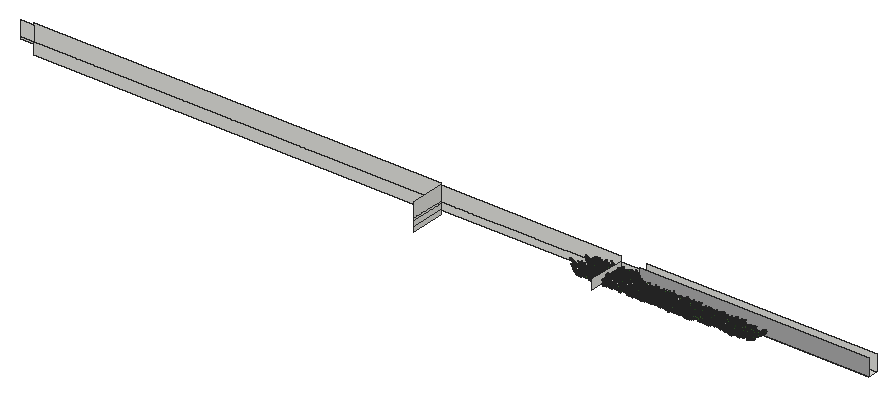
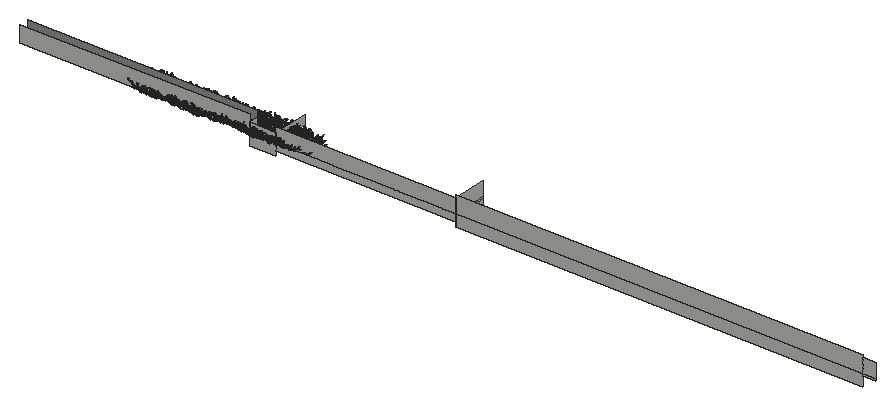
# SketchUp Ruby script. Lengths in inches.
U = 1.inch
M = Sketchup.active_model
def pt(a) = Geom::Point3d.new(a.map { |v| v * U })
def face(e, loops, mat)
  f = e.add_face(loops[0].map { |a| pt(a) })
  loops[1..].each { |l| e.add_face(l.map { |a| pt(a) }).erase! }
  f.material = f.back_material = mat if mat
  f
end
# faces: each face lists its corners as indices into pts; further lists are holes
def faces(e, pts, list, mat = nil) = list.each { |f| face(e, (f[0].is_a?(Array) ? f : [f]).map { |l| l.map { |i| pts[i] } }, mat) }
# xy, xz, yz: faces in a plane at the given z, y or x. An outline is a flat list of corners, or four numbers for a rectangle; further outlines are holes
def ring(l) = l.size == 4 ? [[l[0], l[1]], [l[2], l[1]], [l[2], l[3]], [l[0], l[3]]] : l.each_slice(2).to_a
def flat(e, list, mat, &to3) = list.each { |f| face(e, (f[0].is_a?(Array) ? f : [f]).map { |l| ring(l).map { |u, v| to3.(u, v) } }, mat) }
def xy(e, z, list, mat = nil) = flat(e, list, mat) { |x, y| [x, y, z] }
def xz(e, y, list, mat = nil) = flat(e, list, mat) { |x, z| [x, y, z] }
def yz(e, x, list, mat = nil) = flat(e, list, mat) { |y, z| [x, y, z] }
def lines(e, pts, list) = list.each { |a, b| e.add_line(pt(pts[a]), pt(pts[b])) }
# prism: a flat outline (further loops are holes) pulled along v
def prism(e, loops, v, mat = nil)
  f = face(e, loops, mat); d = Geom::Vector3d.new(v.map { |x| x * U })
  f.pushpull(f.normal.samedirection?(d) ? d.length : -d.length)
end
def box(e, o, s, mat = nil) = prism(e, [[o, [o[0] + s[0], o[1], o[2]], [o[0] + s[0], o[1] + s[1], o[2]], [o[0], o[1] + s[1], o[2]]]], [0, 0, s[2]], mat)
def at(x, y, z, deg = 0) = Geom::Transformation.translation(pt([x, y, z])) * Geom::Transformation.rotation(ORIGIN, Z_AXIS, deg.degrees)
def axes(o, x, y, z) = Geom::Transformation.new([*x, 0, *y, 0, *z, 0, *pt(o).to_a, 1])
def part(name) = M.definitions.add(name)
# library, detail: a bought-in or finely detailed component or shape, given as its bounding box
def library(name, o, s) = part(name).tap { |d| box(d.entities, o, s) }
def detail(e, o, s) = box(e.add_group.entities, o, s)
def put(e, d, t, mat = nil) = e.add_instance(d, t).tap { |i| i.material = mat if mat }
def group(e, t, mat = nil) = e.add_group.tap { |g| g.transformation = t; g.material = mat if mat }.entities
root = M.entities
M.materials.add("Material82").color = [68, 110, 58]
M.materials.add("Material83").color = [48, 90, 38]
M.materials.add("Material84").color = [68, 110, 48]
M.materials.add("Material85").color = [48, 90, 48]
M.materials.add("Material86").color = [58, 110, 58]
M.materials.add("Material87").color = [58, 90, 38]
M.materials.add("Material88").color = [68, 100, 58]
M.materials.add("Material89").color = [48, 100, 38]
M.materials.add("[Color M03]1").color = [170, 170, 170]
c1 = part("grass00")
p = [[-0.6875,0.15,0],[-0.56,0.08,5.52],[-0.04,0.03,2.76],[0.48,-0.02,0],[0.35,-0.02,5.52],[-0.1,-0.14,5.52],
  [-0.12,0.65,8.37],[-0.42,0.65,8.37]]
faces(c1.entities,p,[[0,1,2,3],[3,2,4],[1,5,2],[5,4,2],[1,6,5],[4,5,6],[7,6,1]])
c2 = part("Group16\#1")
put(c2.entities,c1,axes([1.44,-0.61,-0.01],[0.05352,0.12609,0],[-0.10704,0.04543,0.07239],[0.06664,-0.02828,0.11628]),"Material85")
put(c2.entities,c1,axes([0.76,-0.15,-0.01],[0.04676,0.24062,0],[-0.23162,0.04501,0.06642],[0.0652,-0.01267,0.23595]),"Material82")
put(c2.entities,c1,axes([0.79,0.01,-0.01],[-0.00606,0.34651,0],[-0.34381,-0.00602,0.0432],[0.04319,0.00076,0.34386]))
put(c2.entities,c1,axes([1,0.23,-0.01],[-0.07192,0.31144,0],[-0.28722,-0.06632,0.1236],[0.12043,0.02781,0.29478]),"Material84")
put(c2.entities,c1,axes([1.66,0.77,-0.01],[-0.13828,0.29651,0],[-0.21551,-0.1005,0.22471],[0.20365,0.09498,0.23779]),"Material89")
put(c2.entities,c1,axes([0.6875,0.52,-0.01],[-0.18126,0.24051,0],[-0.22746,-0.17142,0.09788],[0.07817,0.05891,0.28481]),"Material84")
put(c2.entities,c1,axes([0.68,0.78,-0.01],[-0.215,0.18688,0],[-0.12385,-0.14248,0.21334],[0.13995,0.16101,0.18878]),"Material82")
put(c2.entities,c1,axes([0.56,1,-0.01],[-0.13756,0.07624,0],[-0.06159,-0.11112,0.0927],[0.04494,0.08108,0.12705]),"Material84")
put(c2.entities,c1,axes([0.2,0.64,-0.01],[-0.23729,0.07254,0],[-0.05711,-0.18681,0.153],[0.04473,0.14632,0.19535]),"Material89")
put(c2.entities,c1,axes([0.0625,0.72,-0.01],[-0.28874,0.02525,0],[-0.02179,-0.24916,0.14647],[0.01276,0.14591,0.25012]),"Material82")
put(c2.entities,c1,axes([-0.08,0.62,-0.01],[-0.34089,-0.04187,0],[0.03255,-0.26504,0.216],[-0.02633,0.21439,0.26703]),"Material89")
put(c2.entities,c1,axes([-0.34,0.98,-0.01],[-0.14314,-0.0493,0],[0.04397,-0.12769,0.06843],[-0.02228,0.0647,0.13505]),"Material89")
put(c2.entities,c1,axes([-0.87,1.45,-0.01],[-0.23488,-0.14114,0],[0.13761,-0.22901,0.06087],[-0.03135,0.05217,0.26717]))
put(c2.entities,c1,axes([-0.72,0.77,-0.01],[-0.14208,-0.13251,0],[0.07209,-0.0773,0.16301],[-0.11118,0.11922,0.1057]),"Material89")
put(c2.entities,c1,axes([-0.62,0.43,-0.01],[-0.14845,-0.21203,0],[0.18654,-0.13061,0.12304],[-0.10079,0.07057,0.22772]),"Material82")
put(c2.entities,c1,axes([-0.68,0.29,-0.01],[-0.13639,-0.32136,0],[0.31723,-0.13464,0.05579],[-0.05136,0.0218,0.34462]),"Material83")
put(c2.entities,c1,axes([-0.64,0.125,-0.01],[-0.0458,-0.23569,0],[0.22124,-0.043,0.08276],[-0.08124,0.01579,0.22538]),"Material86")
put(c2.entities,c1,axes([-1.6,-0.03,-0.01],[0.00576,-0.32897,0],[0.27526,0.00482,0.18018],[-0.18015,-0.00315,0.2753]),"Material84")
put(c2.entities,c1,axes([-1.36,-0.31,-0.01],[0.05718,-0.24765,0],[0.18172,0.04196,0.17267],[-0.16825,-0.03885,0.1865]),"Material89")
put(c2.entities,c1,axes([-1.54,-0.72,-0.01],[0.06537,-0.14017,0],[0.13555,0.06321,0.03939],[-0.0357,-0.01665,0.14956]))
put(c2.entities,c1,axes([-1.19,-0.9,-0.01],[0.09597,-0.12735,0],[0.11214,0.08451,0.07557],[-0.06035,-0.04548,0.14042]),"Material88")
put(c2.entities,c1,axes([-0.47,-0.54,-0.01],[0.11588,-0.10072,0],[0.0618,0.0711,0.12124],[-0.07953,-0.0915,0.0942]))
put(c2.entities,c1,axes([-0.47,-0.84,-0.01],[0.11927,-0.0661,0],[0.06603,0.11913,0.00646],[-0.00313,-0.00565,0.13621]),"Material84")
put(c2.entities,c1,axes([-0.38,-1.24,-0.01],[0.28037,-0.08571,0],[0.0618,0.20215,0.20315],[-0.05939,-0.19428,0.21139]),"Material88")
put(c2.entities,c1,axes([-0.06,-0.66,-0.01],[0.22719,-0.01987,0],[0.01247,0.14255,0.17758],[-0.01547,-0.17691,0.1431]),"Material87")
put(c2.entities,c1,axes([0.11,-0.89,-0.01],[0.14882,0.01828,0],[-0.01058,0.08611,0.12229],[0.01491,-0.12138,0.08676]),"Material85")
put(c2.entities,c1,axes([0.25,-0.72,-0.01],[0.20481,0.07053,0],[-0.06206,0.18022,0.10291],[0.03351,-0.0973,0.1906]),"Material85")
put(c2.entities,c1,axes([0.85,-1.42,-0.01],[0.16481,0.09904,0],[-0.09472,0.15762,0.05616],[0.02893,-0.04814,0.18389]),"Material84")
put(c2.entities,c1,axes([1.01,-1.09,-0.01],[0.21858,0.20385,0],[-0.17495,0.1876,0.15339],[0.10462,-0.11218,0.25652]),"Material89")
put(c2.entities,c1,axes([1.01,-0.71,-0.01],[0.08733,0.12473,0],[-0.06445,0.04512,0.13037],[0.1068,-0.07477,0.07867]),"Material85")
c3 = part("Group15\#1")
put(c3.entities,c2,at(0,0,0))
c4 = part("3darcstudiotree_grass00\#1")
put(c4.entities,c3,at(0,0,0))
xy(root,-34.17,[[1674.99,381.72,1831.09,387.84]])
xz(root,381.72,[[1674.99,-34.17,1831.09,-22.8]],"[Color M03]1")
xz(root,387.84,[[1257.22,-42.1875,1534.73,-34.17],[1657.41,-42.1875,1674.99,-34.17],[1534.73,-39.125,1657.41,-34.17],[1248.34,-35.625,1257.22,-34.17],[1248.34,-34.17,1257.22,-24.25],
  [1257.22,-34.17,1534.73,-22.8],[1534.73,-34.17,1657.41,-24.25],[1657.41,-34.17,1674.99,-27.66],[1674.99,-34.17,1831.09,-22.8]])
yz(root,1534.73,[[364.46,-42.1875,387.84,-39.125],[364.46,-39.125,387.84,-35.625],[364.46,-35.625,387.84,-34.17],[364.46,-34.17,387.84,-24.25]])
yz(root,1657.41,[[362.97,-34.17,387.84,-27.66]])
yz(root,1674.99,[[381.72,-34.17,387.84,-27.66]])
put(root,c4,axes([1646.16,372.86,-34.17],[0.43217,-1.5656,0],[4.20709,0.18062,-0.01362],[0.0661,0.00284,1.54899]))
put(root,c4,axes([1667,373.03,-34.17],[0.37423,-1.77165,0],[3.6892,0.1212,-0.04948],[0.31334,0.01029,1.76318]))
put(root,c4,axes([1660.48,373.13,-34.17],[2.99211,-0.88341,0],[2.54027,1.33816,-0.01707],[0.06311,0.03325,1.96039]))
put(root,c4,axes([1700.4,372.41,-34.17],[-4.26886,-0.01451,0],[0.03771,-1.72573,-0.00939],[0.00047,-0.02147,1.9024]))
put(root,c4,axes([1689.54,372.79,-34.17],[3.91894,1.05311,0],[-2.36552,1.3691,-0.06012],[-0.14517,0.08402,1.3502]))
put(root,c4,axes([1681.87,373.13,-34.17],[3.33812,-0.00931,0],[0.03014,1.68097,-0.0442],[0.00131,0.07293,1.33678]))
put(root,c4,axes([1655.42,373.02,-34.17],[2.55431,1.01117,0],[-3.10398,1.2195,-0.03194],[-0.09397,0.03692,1.36388]))
put(root,c4,axes([1712.625,372.65,-34.17],[-3.78642,0.03695,0],[-0.11198,-1.78455,-0.01248],[-0.00125,-0.01991,1.37214]))
put(root,c4,axes([1744.15,372.82,-34.17],[-3.59063,0.36551,0],[-0.927,-1.41632,-0.03018],[-0.05381,-0.08221,1.98332]))
put(root,c4,axes([1716.72,372.76,-34.17],[-3.89357,0.61481,0],[-1.50479,-1.48217,-0.00598],[-0.01246,-0.01228,1.70205]))
put(root,c4,axes([1679.82,373.3125,-34.17],[-2.43659,-1.39628,0],[3.54139,-0.96116,-0.05298],[0.19991,-0.05426,1.4759]))
put(root,c4,axes([1670.83,373.45,-34.17],[2.25035,1.16277,0],[-2.68664,0.80868,-0.04536],[-0.27393,0.08245,1.92466]))
put(root,c4,axes([1720.54,374.24,-34.17],[0.94723,-1.59052,0],[4.2139,0.39031,-0.04288],[0.2193,0.02031,1.70449]))
put(root,c4,axes([1750.67,374.25,-34.17],[4.40385,0.48107,0],[-1.25638,1.78876,-0.02222],[-0.03253,0.04631,1.93436]))
put(root,c4,axes([1712.65,374.63,-34.17],[0.52677,-1.54843,0],[3.37532,0.17859,-0.00096],[0.0064,0.00034,1.71349]))
put(root,c4,axes([1655.41,374.65,-34.17],[1.00905,-1.48256,0],[4.12419,0.43657,-0.05256],[0.2523,0.02671,1.59089]))
put(root,c4,axes([1717.8125,374.45,-34.17],[-2.54975,-1.13663,0],[2.74994,-0.95943,-0.02762],[0.1264,-0.0441,1.68176]))
put(root,c4,axes([1703.84,374.86,-34.17],[4.10302,-0.30694,0],[0.8385,1.74326,-0.00778],[0.00611,0.0127,1.42033]))
put(root,c4,axes([1677.05,374.0625,-34.17],[-3.06856,1.30795,0],[-2.89535,-1.05647,-0.0352],[-0.142,-0.05181,1.62511]))
put(root,c4,axes([1689.47,374.78,-34.17],[0.60137,-1.69863,0],[3.35822,0.18491,-0.0384],[0.22932,0.01263,1.53253]))
put(root,c4,axes([1732.47,375.0625,-34.17],[3.06207,-0.55792,0],[1.42852,1.21938,-0.0238],[0.07482,0.06387,1.9133]))
put(root,c4,axes([1727.61,374.52,-34.17],[0.41076,1.77313,0],[-3.60416,0.12986,-0.02215],[-0.11578,0.00417,1.42375]))
put(root,c4,axes([1672.28,375.43,-34.17],[-0.12471,-1.80139,0],[4.72201,-0.05084,-0.06757],[0.3331,-0.00359,1.74608]))
put(root,c4,axes([1682.07,374.875,-34.17],[-0.2328,1.40639,0],[-3.78045,-0.09733,-0.01044],[-0.05523,-0.00142,1.50484]))
put(root,c4,axes([1744.24,374.77,-34.17],[-1.9685,1.46825,0],[-4.07305,-0.84931,-0.01892],[-0.07094,-0.01479,1.46501]))
put(root,c4,axes([1661.98,375.07,-34.17],[1.86247,1.54763,0],[-3.42195,0.64048,-0.01135],[-0.06523,0.01221,1.80626]))
put(root,c4,axes([1650.84,375.22,-34.17],[-0.22309,1.29668,0],[-4.38525,-0.11734,-0.00038],[-0.00168,-0.00004,1.44006]))
put(root,c4,axes([1737.04,375.41,-34.17],[1.22817,1.22832,0],[-3.29828,0.51292,-0.04901],[-0.28268,0.04396,1.64754]))
put(root,c4,axes([1697.9375,375.32,-34.17],[-0.96459,1.39728,0],[-4.50708,-0.48391,-0.06593],[-0.29103,-0.03125,1.60187]))
put(root,c4,axes([1696.28,375.42,-34.17],[0.06651,1.49398,0],[-4.62108,0.032,-0.00579],[-0.03066,0.00021,1.83497]))
put(root,c4,axes([1665.18,375.59,-34.17],[-3.98386,-0.59662,0],[1.47731,-1.53422,-0.04397],[0.0965,-0.10022,1.92843]))
put(root,c4,axes([1693.27,376.5,-34.17],[3.81628,-0.13918,0],[0.37321,1.59155,-0.00914],[0.00528,0.02252,1.90465]))
put(root,c4,axes([1664.96,376.41,-34.17],[3.87274,-0.73751,0],[1.55178,1.26734,-0.04306],[0.13654,0.11151,1.95064]))
put(root,c4,axes([1743.24,376.96,-34.17],[4.03419,0.29669,0],[-0.75311,1.59264,-0.00417],[-0.00465,0.00984,1.87295]))
put(root,c4,axes([1705.6,376.69,-34.17],[1.8424,1.14237,0],[-3.65624,0.91712,-0.00074],[-0.00371,0.00093,1.93092]))
put(root,c4,axes([1649.58,376.95,-34.17],[-2.10821,-1.47996,0],[3.50963,-0.77757,-0.0488],[0.18715,-0.04146,1.32723]))
put(root,c4,axes([1738.35,376.96,-34.17],[4.26727,0.66803,0],[-1.41698,1.40776,-0.04113],[-0.07249,0.07202,1.37498]))
put(root,c4,axes([1720.71,377.2,-34.17],[4.15464,-0.59094,0],[1.53872,1.68251,-0.06016],[0.09162,0.10018,1.52593]))
put(root,c4,axes([1716.68,376.61,-34.17],[0.64746,1.71828,0],[-3.59,0.21039,-0.03328],[-0.18561,0.01088,1.53387]))
put(root,c4,axes([1654.41,377.25,-34.17],[2.13524,-1.29449,0],[3.0122,0.77275,-0.01966],[0.10051,0.02579,1.64285]))
put(root,c4,axes([1689.64,376.78,-34.17],[-1.5249,1.25696,0],[-3.62628,-0.68422,-0.02774],[-0.1175,-0.02217,1.41462]))
put(root,c4,axes([1672.08,377.47,-34.17],[3.32502,-0.81851,0],[2.11953,1.33913,-0.03499],[0.11667,0.07371,1.88939]))
put(root,c4,axes([1645.69,376.76,-34.17],[-3.35215,0.96429,0],[-2.54913,-1.37823,-0.03459],[-0.11585,-0.06264,1.84283]))
put(root,c4,axes([1709.41,377.42,-34.17],[-1.38876,-1.54798,0],[3.56891,-0.49797,-0.03351],[0.18812,-0.02625,1.68972]))
put(root,c4,axes([1682.63,376.83,-34.17],[-1.7842,1.38137,0],[-4.14651,-0.83297,-0.01882],[-0.07173,-0.01441,1.49212]))
put(root,c4,axes([1728.79,377.7,-34.17],[0.96466,-1.81909,0],[3.32191,0.27398,-0.01603],[0.09156,0.00755,1.48463]))
put(root,c4,axes([1662.8125,377.27,-34.17],[-2.42169,0.94143,0],[-3.12641,-1.2508,-0.05994],[-0.19111,-0.07646,1.51606]))
put(root,c4,axes([1675.83,377.69,-34.17],[-1.63198,-1.29559,0],[3.66951,-0.7189,-0.01655],[0.08632,-0.01691,1.78815]))
put(root,c4,axes([1734.62,377.29,-34.17],[-1.97144,1.08801,0],[-3.33394,-0.93955,-0.01309],[-0.05439,-0.01533,1.56859]))
put(root,c4,axes([1750.06,377.8,-34.17],[-3.77025,-0.95024,0],[2.35793,-1.45505,-0.05584],[0.17762,-0.10961,1.93872]))
put(root,c4,axes([1700.46,377.51,-34.17],[-0.60649,1.78928,0],[-3.60415,-0.19,-0.04319],[-0.29403,-0.0155,1.87209]))
put(root,c4,axes([1717.27,378.77,-34.17],[2.12492,-1.52639,0],[3.32667,0.72027,-0.02765],[0.13101,0.02837,1.53783]))
put(root,c4,axes([1645.55,378.7,-34.17],[3.10066,0.47843,0],[-1.67535,1.68868,-0.03882],[-0.06401,0.06452,1.55956]))
put(root,c4,axes([1651.15,378.47,-34.17],[2.78968,1.01154,0],[-2.64,1.13236,-0.04265],[-0.18761,0.08047,1.90027]))
put(root,c4,axes([1660.72,378.8,-34.17],[4.11116,0.47333,0],[-1.05643,1.42708,-0.03197],[-0.04362,0.05892,1.37583]))
put(root,c4,axes([1688.89,378.72,-34.17],[3.33503,1.17525,0],[-2.6851,1.18507,-0.00121],[-0.00399,0.00176,1.48985]))
put(root,c4,axes([1722.43,379.08,-34.17],[2.11135,-1.17998,0],[3.12805,0.87051,-0.01427],[0.05324,0.01482,1.30992]))
put(root,c4,axes([1706.38,379,-34.17],[-2.24585,-1.17679,0],[2.75058,-0.81643,-0.02546],[0.1532,-0.04547,1.94365]))
put(root,c4,axes([1728.08,379.3,-34.17],[-1.90322,-1.23489,0],[2.93996,-0.70472,-0.04312],[0.27444,-0.06578,1.92045]))
put(root,c4,axes([1655.09,378.9,-34.17],[-2.52665,1.52426,0],[-3.1276,-0.80632,-0.05029],[-0.29899,-0.07708,1.98932]))
put(root,c4,axes([1699.92,378.94,-34.17],[-1.50368,1.17097,0],[-3.52829,-0.70467,-0.03106],[-0.12382,-0.02473,1.32443]))
put(root,c4,axes([1748.36,379.75,-34.17],[3.38929,-0.88137,0],[2.3631,1.41334,-0.02666],[0.06787,0.04059,1.48784]))
put(root,c4,axes([1711.625,379.73,-34.17],[2.20658,-1.37183,0],[2.86337,0.71632,-0.01781],[0.08885,0.02223,1.50117]))
put(root,c4,axes([1693.3125,379.64,-34.17],[0.14571,-1.35454,0],[4.55175,0.07615,-0.04061],[0.20314,0.0034,1.70991]))
put(root,c4,axes([1738.37,379.53,-34.17],[3.73542,0.56333,0],[-1.36375,1.40645,-0.02441],[-0.06005,0.06193,1.97124]))
put(root,c4,axes([1665.98,379.17,-34.17],[0.11998,1.39847,0],[-4.49149,0.05993,-0.06181],[-0.32467,0.00433,1.77032]))
put(root,c4,axes([1733.68,379.47,-34.17],[2.76774,0.7917,0],[-1.93345,1.05126,-0.02439],[-0.09329,0.05072,1.60766]))
put(root,c4,axes([1672.14,379.76,-34.17],[2.90846,1.13793,0],[-2.61613,1.03996,-0.02475],[-0.10205,0.04057,1.62992]))
put(root,c4,axes([1744.18,379.87,-34.17],[1.66114,1.62878,0],[-3.87747,0.61504,-0.0015],[-0.00686,0.00109,1.54039]))
put(root,c4,axes([1675.9375,379.91,-34.17],[0.65055,1.72425,0],[-3.43127,0.20135,-0.01524],[-0.11013,0.00646,1.90022]))
put(root,c4,axes([1684.6,379.91,-34.17],[-2.50108,0.95556,0],[-2.98511,-1.21518,-0.02879],[-0.10959,-0.04461,1.7592]))
put(root,c4,axes([1737.12,380.69,-34.17],[2.03121,-1.05332,0],[3.7313,1.11909,-0.04371],[0.13933,0.04179,1.40723]))
put(root,c4,axes([1672.25,380.76,-34.17],[4.3644,0.14123,0],[-0.27589,1.32601,-0.01884],[-0.00836,0.04017,1.37151]))
put(root,c4,axes([1656.27,380.67,-34.17],[4.04964,0.85012,0],[-2.04869,1.51784,-0.02998],[-0.08539,0.06326,1.98098]))
put(root,c4,axes([1682.25,380.75,-34.17],[-0.81871,-1.45227,0],[3.80429,-0.33355,-0.01455],[0.06635,-0.00582,1.36448]))
put(root,c4,axes([1717.52,381.01,-34.17],[2.26224,-1.2031,0],[3.43735,1.00525,-0.03781],[0.13632,0.03987,1.4396]))
put(root,c4,axes([1701.85,381.18,-34.17],[3.40778,-1.13854,0],[2.78991,1.29874,-0.02128],[0.06823,0.03176,1.60475]))
put(root,c4,axes([1721.38,380.76,-34.17],[-4.28344,0.1007,0],[-0.25434,-1.68266,-0.00226],[-0.00079,-0.00521,1.87745]))
put(root,c4,axes([1750.39,380.75,-34.17],[-3.53825,1.08299,0],[-2.59336,-1.31776,-0.03049],[-0.10241,-0.05204,1.73706]))
put(root,c4,axes([1660.01,381.41,-34.17],[3.8777,-0.38352,0],[0.80355,1.2636,-0.03452],[0.06321,0.0994,1.86367]))
put(root,c4,axes([1742.95,381.04,-34.17],[-3.68784,-0.24252,0],[0.55953,-1.32329,-0.01602],[0.01459,-0.0345,1.41148]))
put(root,c4,axes([1650.91,381.09,-34.17],[-3.74626,-0.28421,0],[0.67953,-1.39309,-0.01319],[0.01627,-0.03336,1.76124]))
put(root,c4,axes([1706.32,381.61,-34.17],[1.48309,-1.18944,0],[3.17184,0.61511,-0.04022],[0.27217,0.05278,1.99791]))
put(root,c4,axes([1731.82,381.65,-34.17],[3.41982,0.22152,0],[-0.58321,1.40029,-0.00501],[-0.00425,0.0102,1.40942]))
put(root,c4,axes([1665.25,381.62,-34.17],[3.19951,0.37191,0],[-1.24549,1.66647,-0.04213],[-0.05146,0.06886,1.42653]))
put(root,c4,axes([1679.87,381.27,-34.17],[1.18703,1.24458,0],[-3.56072,0.52819,-0.04913],[-0.2933,0.04351,1.81865]))
put(root,c4,axes([1687.63,381.82,-34.17],[4.2261,-0.33522,0],[0.81524,1.59847,-0.02659],[0.0257,0.05039,1.51897]))
put(root,c4,axes([1713.13,381.11,-34.17],[-4.05008,0.95977,0],[-1.76425,-1.15789,-0.02116],[-0.06339,-0.0416,1.49339]))
put(root,c4,axes([1726.19,381.27,-34.17],[-2.75564,1.16599,0],[-3.11928,-1.14656,-0.00031],[-0.00116,-0.00043,1.61707]))
put(root,c4,axes([1694.37,382.22,-34.17],[-4.64372,0.01964,0],[-0.04703,-1.72937,-0.01941],[-0.00122,-0.04491,1.92834]))
put(root,c4,axes([1670.74,382.97,-34.17],[1.86264,-1.28665,0],[3.53883,0.79678,-0.00497],[0.01917,0.00432,1.35772]))
put(root,c4,axes([1684.43,383.25,-34.17],[0.27542,-1.59187,0],[4.66457,0.12552,-0.02398],[0.0893,0.0024,1.30813]))
put(root,c4,axes([1677,382.93,-34.17],[-3.57616,-1.16474,0],[2.7999,-1.33704,-0.02974],[0.0776,-0.03706,1.35064]))
put(root,c4,axes([1707.23,383.33,-34.17],[-1.75334,-1.53625,0],[3.78301,-0.67151,-0.04331],[0.23983,-0.04257,1.88835]))
put(root,c4,axes([1736.76,383.01,-34.17],[-3.93222,-0.02635,0],[0.07503,-1.74154,-0.03595],[0.00307,-0.07126,1.66434]))
put(root,c4,axes([1646.71,383.51,-34.17],[-1.52778,-1.4368,0],[3.26203,-0.53947,-0.00949],[0.054,-0.00893,1.63563]))
put(root,c4,axes([1655.85,383.58,-34.17],[-0.81771,-1.39799,0],[3.86882,-0.35195,-0.03351],[0.1754,-0.01596,1.59864]))
put(root,c4,axes([1734.93,383.74,-34.17],[1.79387,-1.26785,0],[3.18419,0.70071,-0.05199],[0.23586,0.0519,1.41973]))
put(root,c4,axes([1712.03,383.7,-34.17],[-0.47275,-1.4969,0],[4.46074,-0.21911,-0.06365],[0.35527,-0.01745,1.89522]))
put(root,c4,axes([1694.35,383.84,-34.17],[4.39151,-0.30239,0],[0.81207,1.8342,-0.04063],[0.02885,0.06516,1.46079]))
put(root,c4,axes([1688.31,383.8,-34.17],[0.23544,-1.60034,0],[3.90526,0.08936,-0.02273],[0.11635,0.00266,1.50351]))
put(root,c4,axes([1668.29,383.68,-34.17],[4.04452,0.28903,0],[-0.72611,1.58031,-0.0513],[-0.04641,0.10101,1.54883]))
put(root,c4,axes([1745.98,383.49,-34.17],[-2.90199,-1.04001,0],[2.97522,-1.29119,-0.02206],[0.0727,-0.03155,1.62457]))
put(root,c4,axes([1726.54,383.9375,-34.17],[-0.12409,-1.44715,0],[3.33282,-0.04445,-0.02047],[0.13634,-0.00182,1.66543]))
put(root,c4,axes([1700.05,384.15,-34.17],[2.16016,-1.57069,0],[3.42867,0.73339,-0.01711],[0.07383,0.01579,1.43496]))
put(root,c4,axes([1650.5625,383.9375,-34.17],[-1.12016,-1.49158,0],[3.32126,-0.38792,-0.01669],[0.11216,-0.0131,1.82011]))
put(root,c4,axes([1722.25,383.7,-34.17],[0.32393,1.2922,0],[-3.8703,0.1509,-0.01511],[-0.10076,0.00393,1.95375]))
put(root,c4,axes([1662.06,384.33,-34.17],[3.3382,-1.0215,0],[2.0281,1.0308,-0.00126],[0.00417,0.00212,1.3431]))
put(root,c4,axes([1716.76,384.13,-34.17],[-3.07387,-1.37226,0],[2.57369,-0.89663,-0.00245],[0.01347,-0.00469,1.8862]))
put(root,c4,axes([1751.15,384.2,-34.17],[1.42863,1.44478,0],[-4.37041,0.67213,-0.01645],[-0.07678,0.01181,1.76201]))
put(root,c4,axes([1662.78,385.08,-34.17],[1.09339,-1.57965,0],[4.13626,0.44528,-0.00598],[0.02433,0.00262,1.35627]))
put(root,c4,axes([1744.13,385.23,-34.17],[1.06749,-1.46896,0],[3.76494,0.42553,-0.03571],[0.22932,0.02592,1.9611]))
put(root,c4,axes([1677.48,385.49,-34.17],[3.96997,0.02835,0],[-0.08063,1.7564,-0.04973],[-0.00512,0.11159,1.89995]))
put(root,c4,axes([1738.85,385.27,-34.17],[1.59793,1.26945,0],[-3.48077,0.68144,-0.01001],[-0.04528,0.00886,1.4706]))
put(root,c4,axes([1682.83,385.48,-34.17],[-3.18032,-1.25414,0],[2.9494,-1.16324,-0.05204],[0.20858,-0.08226,1.77215]))
put(root,c4,axes([1688.43,385.59,-34.17],[3.671,0.98063,0],[-2.61565,1.5229,-0.02464],[-0.07837,0.04563,1.98292]))
put(root,c4,axes([1721.05,385.83,-34.17],[1.6756,-1.36696,0],[3.5262,0.67226,-0.03335],[0.16368,0.0312,1.60043]))
put(root,c4,axes([1692.9375,386.03,-34.17],[3.22571,-1.00591,0],[2.69072,1.34198,-0.01988],[0.07446,0.03714,1.96304]))
put(root,c4,axes([1750.66,386.04,-34.17],[2.00503,-1.14609,0],[3.00042,0.81639,-0.0362],[0.21042,0.05725,1.92943]))
put(root,c4,axes([1707.38,385.98,-34.17],[-1.47837,-1.71881,0],[3.4357,-0.4596,-0.01224],[0.08437,-0.01129,1.97883]))
put(root,c4,axes([1715.07,386.02,-34.17],[-0.70107,-1.67232,0],[4.13597,-0.26967,-0.0168],[0.0818,-0.00533,1.55067]))
put(root,c4,axes([1655.04,385.5,-34.17],[-2.75278,0.82906,0],[-2.65464,-1.37089,-0.0597],[-0.21369,-0.11035,1.93343]))
put(root,c4,axes([1665.93,385.77,-34.17],[3.04278,1.18912,0],[-3.29647,1.31191,-0.05903],[-0.21773,0.08665,1.83956]))
put(root,c4,axes([1645.66,385.77,-34.17],[-2.50316,1.24796,0],[-3.26881,-1.01974,-0.0328],[-0.10917,-0.03406,1.32564]))
put(root,c4,axes([1671.03,386.54,-34.17],[2.18615,-1.3842,0],[3.44906,0.84721,-0.04551],[0.21226,0.05214,1.67334]))
put(root,c4,axes([1649.16,386.22,-34.17],[-3.58141,-0.41852,0],[1.07572,-1.43168,-0.05017],[0.07746,-0.10309,1.54202]))
put(root,c4,axes([1712.84,386.12,-34.17],[-3.50363,0.54877,0],[-1.37004,-1.36042,-0.04199],[-0.09387,-0.09321,1.68502]))
put(root,c4,axes([1727.41,386.18,-34.17],[1.45904,1.69634,0],[-4.12454,0.55175,-0.04327],[-0.22093,0.02955,1.7601]))
put(root,c4,axes([1699.3,386.58,-34.17],[-1.03876,-1.58927,0],[3.98467,-0.40506,-0.01269],[0.06748,-0.00686,1.69312]))
put(root,c4,axes([1733.92,386.55,-34.17],[3.16719,1.22877,0],[-2.37702,0.9529,-0.00671],[-0.02839,0.01138,1.53359]))
put(root,c4,axes([1661.89,387.62,-34.17],[3.59653,-0.21085,0],[0.631,1.67397,-0.00967],[0.00626,0.01661,1.41667]))
put(root,c4,axes([1715.64,387.57,-34.17],[3.86987,-0.34459,0],[0.79622,1.39073,-0.03599],[0.03867,0.06754,1.32194]))
put(root,c4,axes([1676.55,387.45,-34.17],[2.6716,0.78375,0],[-2.01413,1.06781,-0.0148],[-0.06741,0.03574,1.93047]))
put(root,c4,axes([1744.66,387.2,-34.17],[-3.48173,-0.56284,0],[1.61416,-1.55298,-0.01809],[0.03189,-0.03068,1.4829]))
put(root,c4,axes([1710.03,387.67,-34.17],[-0.94917,-1.78727,0],[4.28932,-0.35429,-0.02019],[0.10216,-0.00844,1.69814]))
put(root,c4,axes([1651.47,387.42,-34.17],[-4.08051,-0.34509,0],[0.80518,-1.48079,-0.03168],[0.03378,-0.06213,1.46389]))
put(root,c4,axes([1721.31,388.1,-34.17],[4.59121,-0.45029,0],[0.84969,1.34743,-0.00031],[0.00049,0.00078,1.72722]))
put(root,c4,axes([1738.14,387.73,-34.17],[-2.98813,-0.54786,0],[1.47052,-1.24742,-0.04575],[0.11826,-0.10032,1.60296]))
put(root,c4,axes([1668.59,387.875,-34.17],[-3.23469,-1.08731,0],[2.23739,-1.03522,-0.02002],[0.06548,-0.0303,1.30322]))
